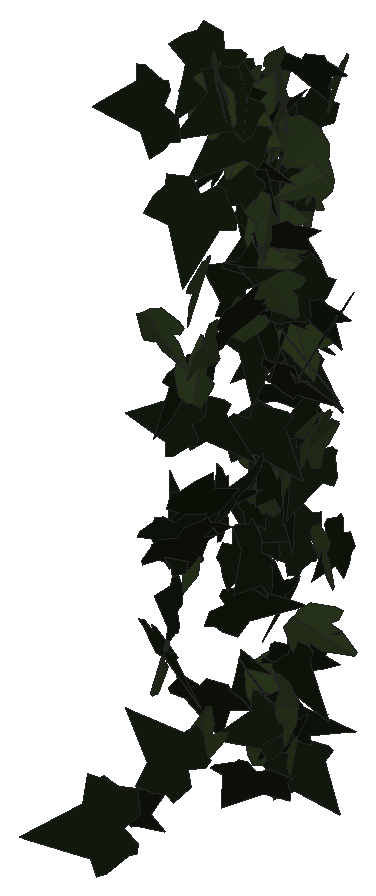
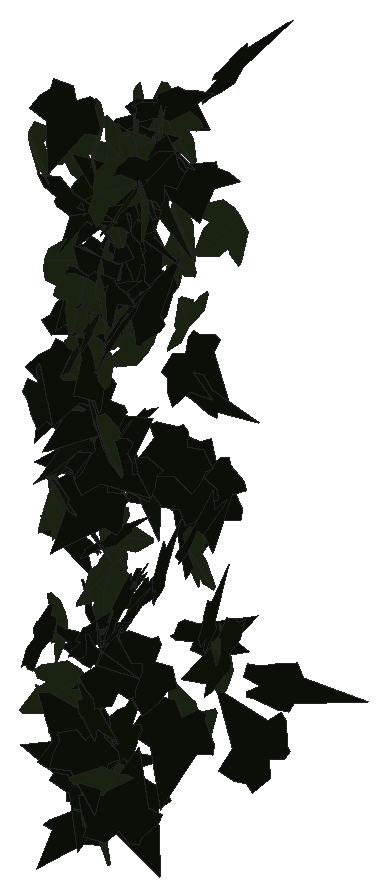
# SketchUp Ruby script. Lengths in inches.
U = 1.inch
M = Sketchup.active_model
def pt(a) = Geom::Point3d.new(a.map { |v| v * U })
def face(e, loops, mat)
  f = e.add_face(loops[0].map { |a| pt(a) })
  loops[1..].each { |l| e.add_face(l.map { |a| pt(a) }).erase! }
  f.material = f.back_material = mat if mat
  f
end
# faces: each face lists its corners as indices into pts; further lists are holes
def faces(e, pts, list, mat = nil) = list.each { |f| face(e, (f[0].is_a?(Array) ? f : [f]).map { |l| l.map { |i| pts[i] } }, mat) }
# xy, xz, yz: faces in a plane at the given z, y or x. An outline is a flat list of corners, or four numbers for a rectangle; further outlines are holes
def ring(l) = l.size == 4 ? [[l[0], l[1]], [l[2], l[1]], [l[2], l[3]], [l[0], l[3]]] : l.each_slice(2).to_a
def flat(e, list, mat, &to3) = list.each { |f| face(e, (f[0].is_a?(Array) ? f : [f]).map { |l| ring(l).map { |u, v| to3.(u, v) } }, mat) }
def xy(e, z, list, mat = nil) = flat(e, list, mat) { |x, y| [x, y, z] }
def xz(e, y, list, mat = nil) = flat(e, list, mat) { |x, z| [x, y, z] }
def yz(e, x, list, mat = nil) = flat(e, list, mat) { |y, z| [x, y, z] }
def lines(e, pts, list) = list.each { |a, b| e.add_line(pt(pts[a]), pt(pts[b])) }
# prism: a flat outline (further loops are holes) pulled along v
def prism(e, loops, v, mat = nil)
  f = face(e, loops, mat); d = Geom::Vector3d.new(v.map { |x| x * U })
  f.pushpull(f.normal.samedirection?(d) ? d.length : -d.length)
end
def box(e, o, s, mat = nil) = prism(e, [[o, [o[0] + s[0], o[1], o[2]], [o[0] + s[0], o[1] + s[1], o[2]], [o[0], o[1] + s[1], o[2]]]], [0, 0, s[2]], mat)
def at(x, y, z, deg = 0) = Geom::Transformation.translation(pt([x, y, z])) * Geom::Transformation.rotation(ORIGIN, Z_AXIS, deg.degrees)
def axes(o, x, y, z) = Geom::Transformation.new([*x, 0, *y, 0, *z, 0, *pt(o).to_a, 1])
def part(name) = M.definitions.add(name)
# library, detail: a bought-in or finely detailed component or shape, given as its bounding box
def library(name, o, s) = part(name).tap { |d| box(d.entities, o, s) }
def detail(e, o, s) = box(e.add_group.entities, o, s)
def put(e, d, t, mat = nil) = e.add_instance(d, t).tap { |i| i.material = mat if mat }
def group(e, t, mat = nil) = e.add_group.tap { |g| g.transformation = t; g.material = mat if mat }.entities
root = M.entities
M.materials.add("efeu1").color = [18, 25, 13]
M.materials.add("efeu2").color = [43, 57, 29]
c1 = part("ivyleaf_9")
p = [[1.54,2.16,1.25],[1.36,2.04,1.19],[-0.21,0.99,0.68],[-0.71,1.11,0.82],[-0.85,0.86,0.67],[-0.8,0.17,0.21],
  [-0.9,-0.01,0.1],[-0.67,-0.16,-0.02],[-0.08,-0.08,-0.05],[-0.03,-0.6,-0.4],[0.65,-0.88,-0.66],[0.83,-0.6,-0.49],
  [1.29,-0.42,-0.43],[1.8125,-0.07,-0.26],[1.21,0.44,0.15]]
faces(c1.entities,p,[[0,1,2,3,4,5,6,7,8,9,10,11,12,13,14]],"efeu1")
c2 = part("ivyleaf_10")
p = [[0,0.5,-0.03],[-0.0625,2.02,-0.43],[-0.19,2.01,-0.46],[-0.54,1.05,-0.29],[-0.52,0.625,-0.18],[-0.83,0.76,-0.28],
  [-1.16,0.64,-0.33],[-1.15,0.33,-0.24],[-0.77,-0.39,0.02],[-0.3,-0.51,0.16],[0.04,-0.48,0.23],[-0.02,2.01,-0.4375],
  [-0.06,2.01,-0.43],[0.04,-0.49,0.23],[0.67,-0.49,0.14],[1.38,0.36,-0.2],[1.375,0.51,-0.24],[0.81,0.65,-0.19],
  [0.62,0.59,-0.15],[0.6,1.09,-0.28],[0.5,1.23,-0.31]]
faces(c2.entities,p,[[0,1,2,3,4,5,6,7,8,9,10],[11,12,0,13,14,15,16,17,18,19,20]],"efeu2")
put(root,c1,axes([597.85,113.5,209.3],[-1.09416,-0.09018,1.0435],[-1.02075,-0.24642,-1.0916],[0.23476,-1.49177,0.11723]))
put(root,c1,axes([599.65,115.89,211.93],[-0.97406,-0.75088,-0.3496],[-0.26844,-0.22436,1.22981],[-0.78357,1.01028,0.01327]))
put(root,c2,axes([597.37,116.52,233.4],[-0.97532,0.22209,-0.70933],[0.69634,-0.13632,-1.00013],[-0.25999,-1.19825,-0.01769]))
put(root,c1,axes([595.17,116.74,208.17],[1.16418,0.25602,-0.50333],[0.45618,0.2534,1.18402],[0.33284,-1.24276,0.13773]))
put(root,c1,axes([595.55,119.3,242.44],[0.30355,-1.14595,-0.77761],[0.20966,-0.74886,1.18544],[-1.36891,-0.36881,0.00913]))
put(root,c2,axes([599.03,118,232.14],[0.00101,-0.88238,-0.79292],[-0.02831,0.79268,-0.88215],[1.18597,0.01968,-0.02038]))
put(root,c1,axes([597.03,118.42,222.23],[0.44029,0.9579,-0.52718],[-0.20921,-0.48401,-1.05419],[-1.07318,0.48734,-0.01078]))
put(root,c2,axes([597.84,119.35,234.87],[0.52016,-1.0802,0.39426],[0.19153,-0.34529,-1.19872],[1.13384,0.55388,0.02161]))
put(root,c1,axes([597.23,118.38,221.5625],[0.44902,1.35526,-0.04667],[-0.019,-0.04287,-1.4277],[-1.35593,0.44939,0.00455]))
put(root,c2,axes([597.95,118.56,229.26],[0.07213,0.95274,-0.69451],[-0.01735,0.69659,0.95379],[1.17887,-0.04805,0.05653]))
put(root,c2,axes([595.54,119.06,213.53],[0.58773,-0.78481,0.74131],[-0.4486,0.59019,0.98048],[-0.98195,-0.73936,-0.00423]))
put(root,c1,axes([596.94,119.55,226.78],[-0.78322,0.32897,0.81601],[-0.76532,0.28421,-0.84914],[-0.43404,-1.09477,0.02476]))
put(root,c2,axes([596.85,120.01,209.92],[-0.33339,-1.21557,0.09661],[0.06888,0.08123,1.25966],[-1.21746,0.33747,0.04481]))
put(root,c1,axes([596.76,120.46,237.72],[-0.73964,-1.12135,-0.34748],[0.18093,0.2969,-1.34326],[1.15992,-0.76135,-0.01205]))
put(root,c1,axes([596.46,120.49,228.99],[-0.22729,0.55334,-1.07617],[0.46504,-0.97097,-0.59746],[-1.11717,-0.51676,-0.02975]))
put(root,c1,axes([594.54,120.19,214.94],[0.94399,-0.87085,0.22516],[0.15845,-0.16029,-1.28429],[0.88542,0.95714,-0.01022]))
put(root,c1,axes([595.07,120.96,216.04],[-0.07556,0.13814,1.11559],[-0.23923,-1.09447,0.11932],[1.09836,-0.22888,0.10273]))
put(root,c1,axes([596.72,119.29,222.4],[0.5744,0.53238,1.11167],[0.84009,0.72836,-0.78288],[-0.90194,1.01746,-0.02123]))
put(root,c1,axes([596.36,120.16,219.76],[-0.3165,-0.95514,0.7801],[0.22072,0.7485,1.00601],[-1.21332,0.38532,-0.02049]))
put(root,c2,axes([596.33,120.42,219.53],[0.26997,-0.2654,-1.16824],[-0.89201,0.75487,-0.37762],[0.79971,0.93159,-0.02683]))
put(root,c1,axes([598.65,119.79,232.08],[0.39731,0.84233,1.09244],[0.42871,1.00515,-0.93094],[-1.31116,0.5839,0.02664]))
put(root,c1,axes([598.57,121.03,223.12],[-0.4052,1.15683,0.49673],[-0.23738,0.44227,-1.22362],[-1.23639,-0.46404,0.07213]))
put(root,c1,axes([595.76,121.875,212],[1.00083,0.68551,-0.53387],[-0.44655,-0.29276,-1.21305],[-0.74535,1.09589,0.00989]))
put(root,c2,axes([595.96,122.49,241.86],[1.13757,0.04284,-0.42704],[-0.42664,-0.01851,-1.13838],[-0.04661,1.21495,-0.00228]))
put(root,c1,axes([597.15,123.17,241.74],[-0.93388,-0.5715,0.59461],[-0.4932,-0.33297,-1.09462],[0.66101,-1.05585,0.02335]))
put(root,c1,axes([597.44,123.08,240.45],[-1.11611,-0.53671,0.2223],[-0.16193,-0.17499,-1.23545],[0.5579,-1.1245,0.08615]))
put(root,c1,axes([595.27,122.1875,225.67],[-0.06599,-0.05628,-1.16381],[0.79063,0.85409,-0.08613],[0.85589,-0.79331,-0.01016]))
put(root,c1,axes([596.72,123.65,231.72],[0.13037,0.16139,1.19378],[-0.73674,-0.93933,0.20745],[0.95309,-0.74818,-0.00293]))
put(root,c1,axes([595.42,123.69,243.18],[-0.86496,-0.90752,0.18303],[-0.10321,-0.15439,-1.2533],[0.92002,-0.87052,0.03147]))
put(root,c2,axes([599.1875,122.69,233.14],[-0.69356,-0.7258,-0.49517],[0.33627,0.36355,-1.00387],[0.81173,-0.77074,-0.00722]))
put(root,c1,axes([598.01,122.83,208.04],[0.27544,0.85581,-0.93751],[-0.70268,-0.69613,-0.84192],[-1.05715,0.6857,0.31536]))
put(root,c2,axes([596.22,122.56,242.25],[-0.67625,0.82142,0.54961],[-0.48232,0.30698,-1.05225],[-0.86265,-0.81556,0.15748]))
put(root,c2,axes([597.15,123.19,240.39],[0.93608,0.79537,-0.30071],[-0.22813,-0.19591,-1.22836],[-0.81914,0.96348,-0.00153]))
put(root,c2,axes([595.95,122.78,242.77],[-0.79258,0.82441,0.15893],[-0.11003,0.11468,-1.1436],[-0.83235,-0.80018,-0.00016]))
put(root,c1,axes([595.17,124.19,219.94],[-0.00457,-0.12447,1.15708],[-0.19015,-1.14146,-0.12354],[1.14812,-0.18954,-0.01586]))
put(root,c1,axes([597.08,124.36,218.17],[-0.08604,-0.78104,0.94094],[-0.07417,-0.9382,-0.78554],[1.22061,-0.11206,0.01859]))
put(root,c2,axes([597.42,122.78,241.98],[0.43897,-0.4453,-1.08934],[-0.4281,1.02258,-0.59052],[1.09622,0.57766,0.2056]))
put(root,c2,axes([597.22,122.81,230.52],[0.03872,-0.83175,0.95346],[-0.03722,0.95274,0.83264],[-1.26472,-0.0535,0.00469]))
put(root,c1,axes([596.59,123.12,218.84],[0.4872,-0.58893,-0.7975],[-0.46393,0.64986,-0.76332],[0.87614,0.6716,0.03928]))
put(root,c1,axes([598.3,124.17,209.99],[-0.64886,-0.30352,0.79751],[-0.67116,-0.43718,-0.71245],[0.52696,-0.93054,0.07458]))
put(root,c1,axes([596.09,123.49,238.69],[-0.94181,0.79963,-0.20285],[0.15466,-0.13126,-1.23548],[-0.81034,-0.95442,-0.00004]))
put(root,c2,axes([599.49,123.42,211.73],[0.44827,-0.4072,-1.07917],[-0.77249,0.75381,-0.60532],[0.85656,0.89293,0.01887]))
put(root,c2,axes([597.45,124.49,235.64],[-0.01759,-0.91105,0.71427],[0.58835,-0.62226,-0.7792],[0.99702,0.35112,0.47241]))
put(root,c1,axes([596.7,124.21,237.15],[-1.0567,0.13155,0.15533],[-0.15428,0.01806,-1.06485],[-0.13278,-1.0679,0.00113]))
put(root,c1,axes([597.1,123.77,225.09],[-0.19488,-0.36891,-1.12579],[0.53721,0.98936,-0.4172],[1.05589,-0.57145,0.00447]))
put(root,c1,axes([597.18,125.03,222.12],[0.01908,-0.66506,0.95638],[0.03865,-0.95562,-0.6653],[1.16425,0.04262,0.00642]))
put(root,c1,axes([596.87,123.9,212.19],[1.02176,-0.26445,-0.33045],[-0.31902,0.08621,-1.05543],[0.27813,1.0704,0.00336]))
put(root,c1,axes([596.41,125.21,232.73],[0.45667,-0.72078,-0.69884],[0.37143,-0.59197,0.85327],[-0.9327,-0.58865,-0.00237]))
put(root,c1,axes([595.96,123.56,215.51],[0.05449,0.51862,-1.1332],[0.18153,1.11888,0.5208],[1.23295,-0.18766,-0.0266]))
put(root,c1,axes([594.49,124.75,240.0625],[0.09382,-0.04199,1.23627],[0.96007,-0.77931,-0.09933],[0.77999,0.96428,-0.02644]))
put(root,c2,axes([599.82,124.47,240.12],[1.02158,-0.0308,-0.7267],[-0.69599,0.32253,-0.99208],[0.21126,1.21148,0.24565]))
put(root,c2,axes([596.83,124.46,240.55],[0.79853,0.04929,0.98333],[-0.98296,-0.03251,0.79985],[0.05632,-1.26631,0.01774]))
put(root,c1,axes([599.05,125.18,231.32],[-0.0385,0.02914,1.21062],[-1.1656,-0.32935,-0.02914],[0.32839,-1.1656,0.0385]))
put(root,c2,axes([596.8125,124.32,235.41],[-0.65007,0.90502,0.30084],[-0.24589,0.19273,-1.11111],[-0.92147,-0.6899,0.08426]))
put(root,c2,axes([597.28,123.8125,208.9],[0.02034,-0.00012,1.14224],[-0.45856,1.04632,0.00827],[-1.04616,-0.45864,0.01858]))
put(root,c2,axes([597.6,125.14,241.89],[-0.47743,0.75238,-0.78133],[0.39718,-0.67311,-0.89087],[-1.00935,-0.62075,0.01902]))
put(root,c2,axes([595.0625,125.28,239.02],[-0.47714,0.40722,-0.91919],[0.49345,-0.79161,-0.60684],[-0.87593,-0.66777,0.15884]))
put(root,c1,axes([598.03,124.74,210.09],[0.6454,-0.18853,1.0595],[1.02639,-0.26347,-0.67211],[0.32344,1.21229,0.0187]))
put(root,c1,axes([595.4,125.09,237.34],[0.5796,-0.43413,0.90897],[0.79209,-0.45147,-0.72069],[0.62232,0.97895,0.07073]))
put(root,c1,axes([598.54,124.29,209.51],[0.23395,1.18942,0.14616],[0.0376,0.14156,-1.21218],[-1.19778,0.23676,-0.0095]))
put(root,c2,axes([597.48,125.38,240.23],[0.5569,-0.95333,0.35906],[0.23365,-0.27876,-1.10254],[0.99154,0.60112,0.05814]))
put(root,c1,axes([597.84,124.41,234.58],[0.91866,0.69872,0.12534],[0.08903,0.08997,-1.15405],[-0.70427,0.92279,0.01761]))
put(root,c2,axes([597,124.75,232.57],[-0.19294,-0.22256,-1.03406],[0.99993,0.30436,-0.25208],[0.34489,-1.00691,0.15236]))
put(root,c1,axes([594.85,125.32,241.18],[-0.24059,-1.01985,-0.55151],[0.20681,0.51648,-1.04528],[1.14083,-0.3087,0.07318]))
put(root,c2,axes([596.9,125.1,222.23],[-0.10822,0.07122,-1.061],[-1.04244,0.20355,0.11999],[0.21005,1.0469,0.04885]))
put(root,c1,axes([595.61,125.49,237.37],[-0.11846,-0.10515,-1.16065],[1.1471,0.19545,-0.13479],[0.20575,-1.15019,0.0832]))
put(root,c2,axes([596.08,124.37,240.66],[-0.07052,0.41004,1.10293],[-0.15575,1.09193,-0.41591],[-1.16633,-0.1706,-0.01115]))
put(root,c1,axes([595.72,126.19,218.46],[-0.02001,-0.98467,0.67121],[-0.02417,-0.67083,-0.98484],[1.19143,-0.03015,-0.00871]))
put(root,c1,axes([596.35,125.48,214.94],[0.58451,0.70579,0.55943],[-0.35883,-0.4292,0.9164],[0.82604,-0.68586,0.00222]))
put(root,c2,axes([596.99,125.43,238.91],[-0.95916,-0.49863,0.44577],[-0.39908,-0.19875,-1.081],[0.53673,-1.03885,-0.00715]))
put(root,c2,axes([597.37,125.16,233.6],[-0.99779,-0.38172,-0.40446],[0.37223,0.15888,-1.06821],[0.41321,-1.06486,-0.01439]))
put(root,c1,axes([596.08,124.88,238.75],[0.33781,1.08296,-0.16381],[0.02064,0.1651,1.13405],[1.09508,-0.33719,0.02915]))
put(root,c1,axes([597.7,125.71,212.44],[0.05676,-0.27807,-1.22493],[1.21128,0.33674,-0.02031],[0.33255,-1.17911,0.28308]))
put(root,c2,axes([596.9375,125.26,234.65],[0.75494,0.80094,0.31522],[0.1923,0.25175,-1.1002],[-0.83898,0.77841,0.03147]))
put(root,c1,axes([595.54,126.13,228.01],[0.03293,-1.17597,0.1897],[-0.02745,-0.19047,-1.17598],[1.19085,0.02813,-0.03235]))
put(root,c1,axes([595.51,126.28,238.91],[0.13458,-0.89301,0.59242],[0.15224,-0.57509,-0.90147],[1.06078,0.19583,0.05421]))
put(root,c2,axes([597.71,125.51,208.72],[0.94027,-0.67287,-0.48666],[-0.36253,0.32881,-1.15506],[0.74711,1.00639,0.052]))
put(root,c1,axes([598.2,125.4,207.78],[0.05832,-0.64691,-0.92869],[0.17239,0.92415,-0.63292],[1.11859,-0.10869,0.14596]))
put(root,c1,axes([596.34,125.55,234.27],[-0.43528,-0.2475,1.05029],[1.00956,0.30648,0.49062],[-0.38101,1.09483,0.10009]))
put(root,c1,axes([596.37,126.77,234.57],[-0.51712,-0.90918,0.34186],[-0.12815,-0.32004,-1.04501],[0.96284,-0.5309,0.04451]))
put(root,c1,axes([596.75,125.9,226.33],[0.89543,-0.19402,0.66311],[0.65354,-0.11428,-0.91595],[0.22413,1.10835,0.02164]))
put(root,c1,axes([595.62,125.6,220.29],[0.57494,-0.48773,-0.98454],[-0.74702,0.64132,-0.75394],[0.8057,0.94265,0.00353]))
put(root,c1,axes([595.8,126.89,223.07],[-0.35913,-1.04313,0.34089],[0.05014,-0.3739,-1.09132],[1.09627,-0.32462,0.16158]))
put(root,c2,axes([598.57,125.77,214.54],[-0.71681,-0.28568,-1.00092],[0.95525,0.3022,-0.77036],[0.41347,-1.19346,0.04452]))
put(root,c1,axes([595.48,126.04,233.44],[0.61222,-0.79634,-0.50815],[-0.32074,0.39433,-1.0044],[0.88854,0.69104,-0.01243]))
put(root,c1,axes([596.17,125.92,227.15],[0.17525,-0.23641,1.17944],[-0.77935,0.88558,0.29331],[-0.91629,-0.79845,-0.0239]))
put(root,c1,axes([598.47,125.71,242.92],[0.89784,0.56934,-0.29116],[-0.24536,-0.15675,-1.06314],[-0.59053,0.93077,-0.00095]))
put(root,c1,axes([596.1875,125.9,239.26],[0.14046,-0.6804,-0.8475],[-0.05512,0.84899,-0.69073],[1.08543,0.13116,0.0746]))
put(root,c1,axes([596.79,126.63,229.29],[-0.67556,0.23001,-0.82515],[0.77832,-0.27407,-0.71362],[-0.35776,-1.0306,0.00562]))
put(root,c1,axes([595.19,126.74,209.11],[0.89651,0.24409,0.77946],[-0.74929,-0.21489,0.92911],[0.32511,-1.16838,-0.00805]))
put(root,c1,axes([598.37,126.78,222.65],[-1.04687,-0.2994,-0.37019],[0.35475,0.10588,-1.08883],[0.31755,-1.10533,-0.00403]))
put(root,c2,axes([596.32,126.35,220.78],[-0.1958,-1.16254,-0.2124],[0.0699,0.20353,-1.17841],[1.17971,-0.20501,0.03457]))
put(root,c1,axes([597.24,126.29,211.99],[0.95265,0.74399,-0.18717],[0.1474,0.11536,1.20875],[0.75288,-0.96399,0.00019]))
put(root,c2,axes([596.82,126.36,231.59],[-0.81444,-0.01341,-0.69813],[0.69773,-0.05732,-0.81287],[-0.02714,-1.07118,0.05224]))
put(root,c2,axes([598.35,126.86,218.09],[-0.4937,0.47605,-0.95253],[0.6466,-0.70018,-0.68507],[-0.84607,-0.81289,0.03226]))
put(root,c2,axes([598.4,126.95,224.1],[0.14688,-1.0352,0.39436],[0.02378,-0.39477,-1.04515],[1.10752,0.14577,-0.02985]))
put(root,c2,axes([596.26,125.76,221.12],[0.07246,-0.47808,-1.15184],[0.31001,1.12448,-0.44722],[1.20797,-0.25991,0.18386]))
put(root,c1,axes([596.36,126.15,229.24],[1.18863,0.16686,0.16905],[0.15976,0.07676,-1.1991],[-0.17577,1.19813,0.05328]))
put(root,c1,axes([597.01,126.375,239.49],[0.96901,-0.27585,-0.4644],[-0.45237,0.10675,-1.00732],[0.29516,1.06923,-0.01925]))
put(root,c2,axes([598.06,127.4,236.08],[-0.20453,-0.09458,1.05284],[-0.24129,-1.03988,-0.14029],[1.02917,-0.26259,0.17634]))
put(root,c1,axes([596.52,127.0625,235.625],[-1.00967,-0.48929,-0.54058],[0.48352,0.2418,-1.12196],[0.54575,-1.11946,-0.00607]))
put(root,c1,axes([598.14,126.1875,230.29],[1.07951,0.50605,-0.24222],[-0.22671,-0.08697,-1.19211],[-0.51318,1.10292,0.01713]))
put(root,c2,axes([597.46,126.54,228.29],[0.95655,0.39528,0.38425],[0.28169,0.31102,-1.02118],[-0.47387,0.98281,0.16861]))
put(root,c1,axes([596.71,127.64,232.23],[0.09313,-0.79028,0.87266],[0.16586,-0.85785,-0.79456],[1.16558,0.18521,0.04333]))
put(root,c1,axes([596.3125,127.25,219.64],[-0.1908,-0.19871,-0.97712],[0.99414,-0.11479,-0.17078],[-0.07705,-0.98894,0.21616]))
put(root,c1,axes([597.17,126.56,212.43],[0.19737,0.94279,-0.38811],[-0.11904,-0.3713,-0.9625],[-1.01258,0.22742,0.03751]))
put(root,c2,axes([595.86,126.47,210.99],[0.62744,0.88081,0.55524],[0.3138,0.45816,-1.08139],[-0.9928,0.70147,0.00911]))
put(root,c1,axes([596.02,127.32,227.33],[0.04636,0.2626,-1.04836],[-0.23267,-1.02229,-0.26636],[-1.05541,0.23691,0.01267]))
put(root,c2,axes([596.27,126.6875,235.74],[-0.63481,0.9004,0.31517],[-0.48321,0.02292,-1.03876],[-0.82253,-0.70837,0.367]))
put(root,c1,axes([596.33,127.82,218.29],[-0.35778,-0.56592,0.747],[-0.37677,-0.64526,-0.6693],[0.85809,-0.51928,0.01758]))
put(root,c2,axes([595.39,127.81,240.62],[0.00967,0.34776,-1.11875],[-0.29268,-1.08259,-0.33905],[-1.1344,0.28228,0.07794]))
put(root,c2,axes([598.84,126.15,223.43],[0.14217,0.02874,1.16035],[-0.5313,1.04098,0.03931],[-1.03197,-0.53197,0.13962]))
put(root,c1,axes([596.58,127.38,215.08],[-0.69574,0.30135,-0.64507],[0.51655,-0.40708,-0.74729],[-0.49001,-0.85701,0.12813]))
put(root,c1,axes([598.04,126.95,224.64],[-0.96937,0.71414,0.09077],[-0.07253,0.05459,-1.20403],[-0.71622,-0.97208,-0.00093]))
put(root,c1,axes([596.84,126.95,227.58],[1.03442,-0.45759,-0.01349],[-0.01002,0.01069,-1.1311],[0.45768,1.03446,0.00572]))
put(root,c1,axes([599.125,127.31,229.58],[-0.7303,0.6995,-0.61766],[0.38557,-0.48805,-1.0086],[-0.84979,-0.82259,0.07318]))
put(root,c1,axes([597.15,127.08,227.05],[0.72133,-0.79795,-0.19965],[0.04123,0.30029,-1.05121],[0.82152,0.68557,0.22806]))
put(root,c1,axes([597.375,127.29,217.59],[-0.89092,0.23861,0.66627],[-0.65223,0.13889,-0.92189],[-0.27466,-1.10379,0.02803]))
put(root,c1,axes([598.23,127.04,239.01],[-0.55039,0.39051,0.93386],[-0.83233,0.43033,-0.6705],[-0.57604,-0.9949,0.07654]))
put(root,c2,axes([595.87,127.06,228.45],[0.61053,-0.35892,-0.83766],[-0.65261,0.53156,-0.70341],[0.63608,0.88987,0.08232]))
put(root,c1,axes([595.98,126.78,225.18],[0.9982,0.59269,0.15764],[0.14973,0.05652,-1.16057],[-0.59474,1.00899,-0.02759]))
put(root,c1,axes([598.5625,128.25,217.88],[0.12564,-0.2917,-1.02147],[0.69445,-0.75582,0.30125],[-0.80388,-0.69851,0.10059]))
put(root,c2,axes([596.86,127.32,235.14],[-1.03753,0.09397,-0.02768],[0.02739,-0.00452,-1.04178],[-0.09406,-1.03789,0.00203]))
put(root,c1,axes([596.65,126.57,230.8],[0.04864,0.46043,1.06286],[0.04792,1.06209,-0.46229],[-1.15732,0.06333,0.02553]))
put(root,c2,axes([598.91,127.83,241.82],[0.47743,-0.92452,0.24382],[0.08993,-0.22789,-1.04024],[0.95189,0.48523,-0.02401]))
